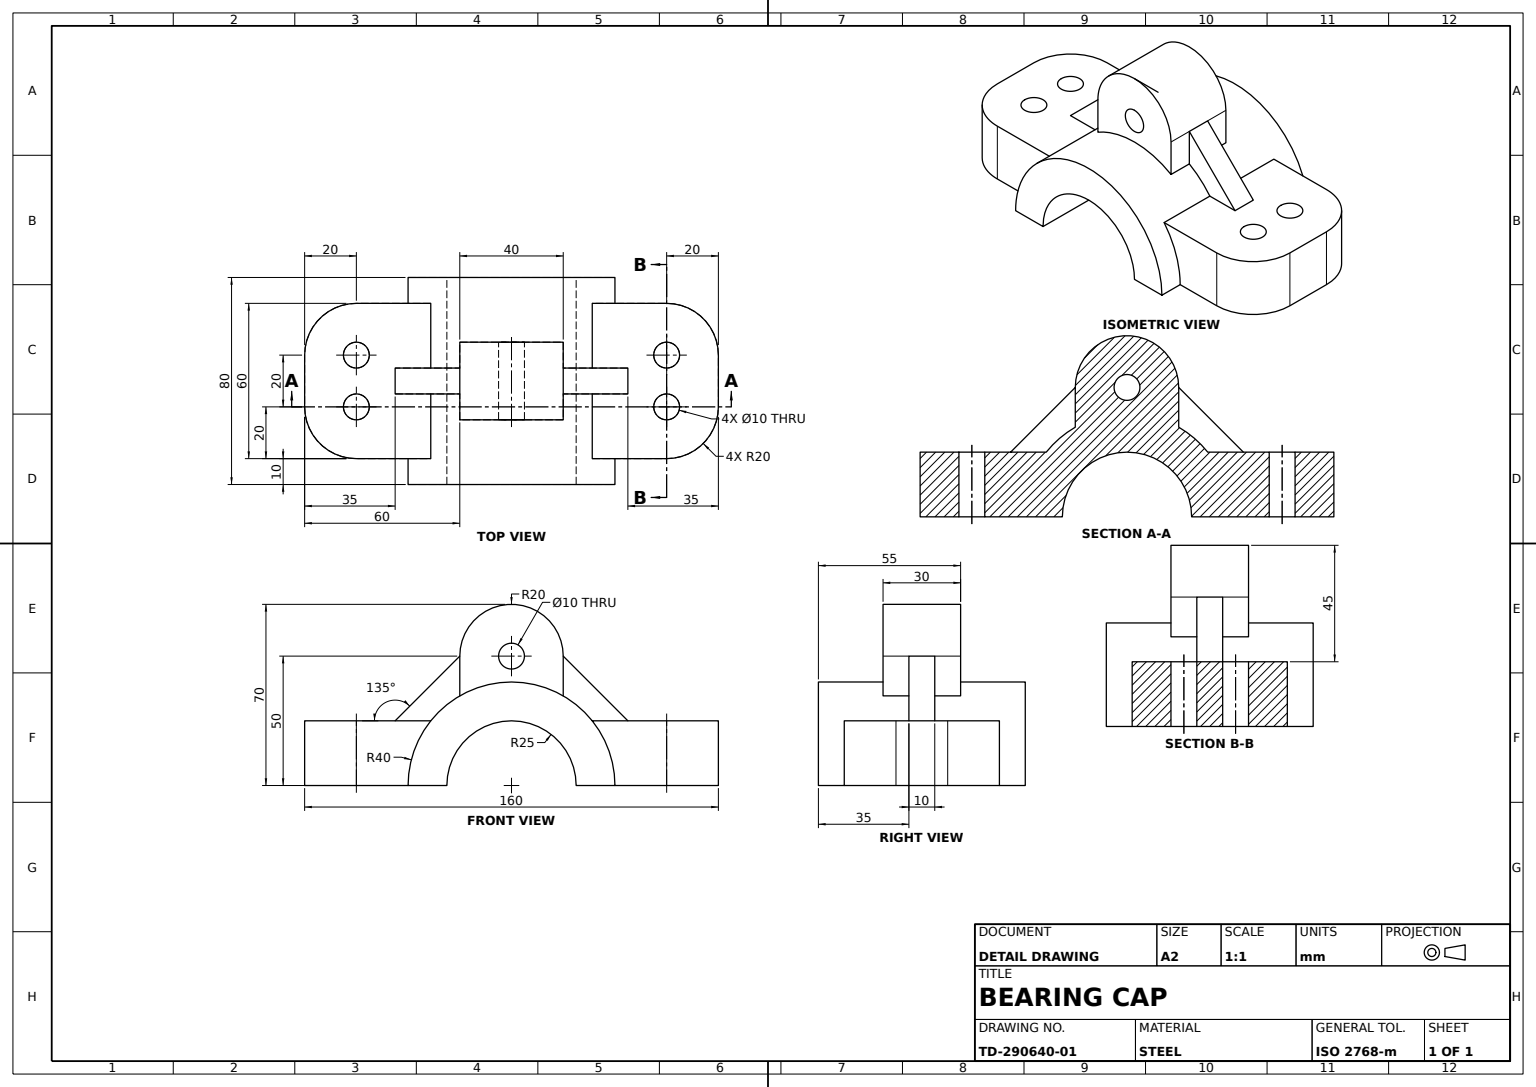
ISO-10303-21;
HEADER;
FILE_DESCRIPTION((''),'2;1');
FILE_NAME('','',(''),(''),'','','');
FILE_SCHEMA(('AUTOMOTIVE_DESIGN'));
ENDSEC;
DATA;
#1=APPLICATION_CONTEXT('');
#2=PRODUCT_CONTEXT('',#1,'mechanical');
#3=PRODUCT('','','',(#2));
#4=PRODUCT_DEFINITION_FORMATION('','',#3);
#5=PRODUCT_DEFINITION_CONTEXT('',#1,'design');
#6=PRODUCT_DEFINITION('','',#4,#5);
#7=PRODUCT_DEFINITION_SHAPE('','',#6);
#8=(LENGTH_UNIT()NAMED_UNIT(*)SI_UNIT(.MILLI.,.METRE.));
#9=(NAMED_UNIT(*)PLANE_ANGLE_UNIT()SI_UNIT($,.RADIAN.));
#10=(NAMED_UNIT(*)SI_UNIT($,.STERADIAN.)SOLID_ANGLE_UNIT());
#11=UNCERTAINTY_MEASURE_WITH_UNIT(LENGTH_MEASURE(0.005),#8,'distance_accuracy_value','');
#12=(GEOMETRIC_REPRESENTATION_CONTEXT(3)GLOBAL_UNCERTAINTY_ASSIGNED_CONTEXT((#11))GLOBAL_UNIT_ASSIGNED_CONTEXT((#8,#9,#10))REPRESENTATION_CONTEXT('',''));
#13=CARTESIAN_POINT('',(80.,10.,25.));
#14=VERTEX_POINT('',#13);
#15=CARTESIAN_POINT('',(60.,30.,25.));
#16=VERTEX_POINT('',#15);
#17=CARTESIAN_POINT('',(60.,10.,25.));
#18=DIRECTION('',(0.,0.,1.));
#19=DIRECTION('',(1.,0.,0.));
#20=AXIS2_PLACEMENT_3D('',#17,#18,#19);
#21=CIRCLE('',#20,20.);
#22=EDGE_CURVE('',#14,#16,#21,.T.);
#23=ORIENTED_EDGE('',*,*,#22,.F.);
#24=CARTESIAN_POINT('',(80.,10.,0.));
#25=VERTEX_POINT('',#24);
#26=DIRECTION('',(0.,0.,-1.));
#27=VECTOR('',#26,1000.);
#28=LINE('',#13,#27);
#29=EDGE_CURVE('',#25,#14,#28,.F.);
#30=ORIENTED_EDGE('',*,*,#29,.F.);
#31=CARTESIAN_POINT('',(60.,30.,0.));
#32=VERTEX_POINT('',#31);
#33=CARTESIAN_POINT('',(60.,10.,0.));
#34=AXIS2_PLACEMENT_3D('',#33,#18,#19);
#35=CIRCLE('',#34,20.);
#36=EDGE_CURVE('',#32,#25,#35,.F.);
#37=ORIENTED_EDGE('',*,*,#36,.F.);
#38=LINE('',#15,#27);
#39=EDGE_CURVE('',#16,#32,#38,.T.);
#40=ORIENTED_EDGE('',*,*,#39,.F.);
#41=EDGE_LOOP('',(#23,#30,#37,#40));
#42=FACE_BOUND('',#41,.T.);
#43=DIRECTION('',(-1.,0.,0.));
#44=AXIS2_PLACEMENT_3D('',#17,#26,#43);
#45=CYLINDRICAL_SURFACE('',#44,20.);
#46=ADVANCED_FACE('',(#42),#45,.T.);
#47=CARTESIAN_POINT('',(-55.,10.,0.));
#48=VERTEX_POINT('',#47);
#49=CARTESIAN_POINT('',(-60.,10.,0.));
#50=AXIS2_PLACEMENT_3D('',#49,#18,#19);
#51=CIRCLE('',#50,5.);
#52=EDGE_CURVE('',#48,#48,#51,.T.);
#53=ORIENTED_EDGE('',*,*,#52,.F.);
#54=EDGE_LOOP('',(#53));
#55=FACE_BOUND('',#54,.T.);
#56=CARTESIAN_POINT('',(-65.,10.,25.));
#57=VERTEX_POINT('',#56);
#58=CARTESIAN_POINT('',(-60.,10.,25.));
#59=AXIS2_PLACEMENT_3D('',#58,#26,#43);
#60=CIRCLE('',#59,5.);
#61=EDGE_CURVE('',#57,#57,#60,.T.);
#62=ORIENTED_EDGE('',*,*,#61,.F.);
#63=EDGE_LOOP('',(#62));
#64=FACE_BOUND('',#63,.T.);
#65=CYLINDRICAL_SURFACE('',#59,5.);
#66=ADVANCED_FACE('',(#55,#64),#65,.F.);
#67=CARTESIAN_POINT('',(-20.,15.,50.));
#68=VERTEX_POINT('',#67);
#69=CARTESIAN_POINT('',(-20.,15.,34.641016));
#70=VERTEX_POINT('',#69);
#71=LINE('',#67,#27);
#72=EDGE_CURVE('',#68,#70,#71,.T.);
#73=ORIENTED_EDGE('',*,*,#72,.T.);
#74=CARTESIAN_POINT('',(-20.,5.,34.641016));
#75=VERTEX_POINT('',#74);
#76=CARTESIAN_POINT('',(-20.,-40.,34.641016));
#77=DIRECTION('',(0.,1.,0.));
#78=VECTOR('',#77,1000.);
#79=LINE('',#76,#78);
#80=EDGE_CURVE('',#70,#75,#79,.F.);
#81=ORIENTED_EDGE('',*,*,#80,.T.);
#82=CARTESIAN_POINT('',(-20.,5.,50.));
#83=VERTEX_POINT('',#82);
#84=CARTESIAN_POINT('',(-20.,5.,0.));
#85=VECTOR('',#18,1000.);
#86=LINE('',#84,#85);
#87=EDGE_CURVE('',#75,#83,#86,.T.);
#88=ORIENTED_EDGE('',*,*,#87,.T.);
#89=CARTESIAN_POINT('',(-20.,-15.,50.));
#90=LINE('',#89,#78);
#91=EDGE_CURVE('',#83,#68,#90,.T.);
#92=ORIENTED_EDGE('',*,*,#91,.T.);
#93=EDGE_LOOP('',(#73,#81,#88,#92));
#94=FACE_BOUND('',#93,.T.);
#95=AXIS2_PLACEMENT_3D('',#89,#19,#26);
#96=PLANE('',#95);
#97=ADVANCED_FACE('',(#94),#96,.F.);
#98=CARTESIAN_POINT('',(45.,5.,25.));
#99=VERTEX_POINT('',#98);
#100=CARTESIAN_POINT('',(31.22499,5.,25.));
#101=VERTEX_POINT('',#100);
#102=CARTESIAN_POINT('',(0.,5.,25.));
#103=VECTOR('',#43,1000.);
#104=LINE('',#102,#103);
#105=EDGE_CURVE('',#99,#101,#104,.T.);
#106=ORIENTED_EDGE('',*,*,#105,.T.);
#107=CARTESIAN_POINT('',(20.,5.,34.641016));
#108=VERTEX_POINT('',#107);
#109=CARTESIAN_POINT('',(0.,5.,0.));
#110=AXIS2_PLACEMENT_3D('',#109,#77,#18);
#111=CIRCLE('',#110,40.);
#112=EDGE_CURVE('',#108,#101,#111,.T.);
#113=ORIENTED_EDGE('',*,*,#112,.F.);
#114=CARTESIAN_POINT('',(20.,5.,50.));
#115=VERTEX_POINT('',#114);
#116=CARTESIAN_POINT('',(20.,5.,0.));
#117=LINE('',#116,#85);
#118=EDGE_CURVE('',#108,#115,#117,.T.);
#119=ORIENTED_EDGE('',*,*,#118,.T.);
#120=DIRECTION('',(0.707106781,0.,-0.707106781));
#121=VECTOR('',#120,1000.);
#122=LINE('',#114,#121);
#123=EDGE_CURVE('',#115,#99,#122,.T.);
#124=ORIENTED_EDGE('',*,*,#123,.T.);
#125=EDGE_LOOP('',(#106,#113,#119,#124));
#126=FACE_BOUND('',#125,.T.);
#127=PLANE('',#110);
#128=ADVANCED_FACE('',(#126),#127,.T.);
#129=CARTESIAN_POINT('',(-65.,-10.,25.));
#130=VERTEX_POINT('',#129);
#131=CARTESIAN_POINT('',(-60.,-10.,25.));
#132=AXIS2_PLACEMENT_3D('',#131,#26,#43);
#133=CIRCLE('',#132,5.);
#134=EDGE_CURVE('',#130,#130,#133,.T.);
#135=ORIENTED_EDGE('',*,*,#134,.F.);
#136=EDGE_LOOP('',(#135));
#137=FACE_BOUND('',#136,.T.);
#138=CARTESIAN_POINT('',(-55.,-10.,0.));
#139=VERTEX_POINT('',#138);
#140=CARTESIAN_POINT('',(-60.,-10.,0.));
#141=AXIS2_PLACEMENT_3D('',#140,#18,#19);
#142=CIRCLE('',#141,5.);
#143=EDGE_CURVE('',#139,#139,#142,.T.);
#144=ORIENTED_EDGE('',*,*,#143,.F.);
#145=EDGE_LOOP('',(#144));
#146=FACE_BOUND('',#145,.T.);
#147=CYLINDRICAL_SURFACE('',#132,5.);
#148=ADVANCED_FACE('',(#137,#146),#147,.F.);
#149=CARTESIAN_POINT('',(-45.,5.,25.));
#150=VERTEX_POINT('',#149);
#151=CARTESIAN_POINT('',(-31.22499,5.,25.));
#152=VERTEX_POINT('',#151);
#153=VECTOR('',#19,1000.);
#154=LINE('',#102,#153);
#155=EDGE_CURVE('',#150,#152,#154,.T.);
#156=ORIENTED_EDGE('',*,*,#155,.F.);
#157=DIRECTION('',(-0.707106781,0.,-0.707106781));
#158=VECTOR('',#157,1000.);
#159=LINE('',#82,#158);
#160=EDGE_CURVE('',#83,#150,#159,.T.);
#161=ORIENTED_EDGE('',*,*,#160,.F.);
#162=ORIENTED_EDGE('',*,*,#87,.F.);
#163=DIRECTION('',(0.,-1.,0.));
#164=AXIS2_PLACEMENT_3D('',#109,#163,#26);
#165=CIRCLE('',#164,40.);
#166=EDGE_CURVE('',#75,#152,#165,.T.);
#167=ORIENTED_EDGE('',*,*,#166,.T.);
#168=EDGE_LOOP('',(#156,#161,#162,#167));
#169=FACE_BOUND('',#168,.T.);
#170=PLANE('',#164);
#171=ADVANCED_FACE('',(#169),#170,.F.);
#172=CARTESIAN_POINT('',(25.,40.,0.));
#173=VERTEX_POINT('',#172);
#174=CARTESIAN_POINT('',(40.,40.,0.));
#175=VERTEX_POINT('',#174);
#176=CARTESIAN_POINT('',(0.,40.,0.));
#177=LINE('',#176,#153);
#178=EDGE_CURVE('',#173,#175,#177,.T.);
#179=ORIENTED_EDGE('',*,*,#178,.F.);
#180=CARTESIAN_POINT('',(-25.,40.,0.));
#181=VERTEX_POINT('',#180);
#182=AXIS2_PLACEMENT_3D('',#176,#163,#26);
#183=CIRCLE('',#182,25.);
#184=EDGE_CURVE('',#173,#181,#183,.T.);
#185=ORIENTED_EDGE('',*,*,#184,.T.);
#186=CARTESIAN_POINT('',(-40.,40.,0.));
#187=VERTEX_POINT('',#186);
#188=EDGE_CURVE('',#187,#181,#177,.T.);
#189=ORIENTED_EDGE('',*,*,#188,.F.);
#190=AXIS2_PLACEMENT_3D('',#176,#163,#19);
#191=CIRCLE('',#190,40.);
#192=EDGE_CURVE('',#175,#187,#191,.T.);
#193=ORIENTED_EDGE('',*,*,#192,.F.);
#194=EDGE_LOOP('',(#179,#185,#189,#193));
#195=FACE_BOUND('',#194,.T.);
#196=PLANE('',#182);
#197=ADVANCED_FACE('',(#195),#196,.F.);
#198=CARTESIAN_POINT('',(80.,-10.,0.));
#199=VERTEX_POINT('',#198);
#200=CARTESIAN_POINT('',(60.,-30.,0.));
#201=VERTEX_POINT('',#200);
#202=CARTESIAN_POINT('',(60.,-10.,0.));
#203=AXIS2_PLACEMENT_3D('',#202,#18,#19);
#204=CIRCLE('',#203,20.);
#205=EDGE_CURVE('',#199,#201,#204,.F.);
#206=ORIENTED_EDGE('',*,*,#205,.F.);
#207=CARTESIAN_POINT('',(80.,-10.,25.));
#208=VERTEX_POINT('',#207);
#209=LINE('',#207,#27);
#210=EDGE_CURVE('',#208,#199,#209,.T.);
#211=ORIENTED_EDGE('',*,*,#210,.F.);
#212=CARTESIAN_POINT('',(60.,-30.,25.));
#213=VERTEX_POINT('',#212);
#214=CARTESIAN_POINT('',(60.,-10.,25.));
#215=AXIS2_PLACEMENT_3D('',#214,#18,#19);
#216=CIRCLE('',#215,20.);
#217=EDGE_CURVE('',#213,#208,#216,.T.);
#218=ORIENTED_EDGE('',*,*,#217,.F.);
#219=LINE('',#212,#27);
#220=EDGE_CURVE('',#201,#213,#219,.F.);
#221=ORIENTED_EDGE('',*,*,#220,.F.);
#222=EDGE_LOOP('',(#206,#211,#218,#221));
#223=FACE_BOUND('',#222,.T.);
#224=AXIS2_PLACEMENT_3D('',#214,#26,#43);
#225=CYLINDRICAL_SURFACE('',#224,20.);
#226=ADVANCED_FACE('',(#223),#225,.T.);
#227=ORIENTED_EDGE('',*,*,#61,.T.);
#228=EDGE_LOOP('',(#227));
#229=FACE_BOUND('',#228,.T.);
#230=ORIENTED_EDGE('',*,*,#134,.T.);
#231=EDGE_LOOP('',(#230));
#232=FACE_BOUND('',#231,.T.);
#233=CARTESIAN_POINT('',(-80.,10.,25.));
#234=VERTEX_POINT('',#233);
#235=CARTESIAN_POINT('',(-80.,-10.,25.));
#236=VERTEX_POINT('',#235);
#237=CARTESIAN_POINT('',(-80.,30.,25.));
#238=VECTOR('',#163,1000.);
#239=LINE('',#237,#238);
#240=EDGE_CURVE('',#234,#236,#239,.T.);
#241=ORIENTED_EDGE('',*,*,#240,.T.);
#242=CARTESIAN_POINT('',(-60.,-30.,25.));
#243=VERTEX_POINT('',#242);
#244=AXIS2_PLACEMENT_3D('',#131,#18,#19);
#245=CIRCLE('',#244,20.);
#246=EDGE_CURVE('',#236,#243,#245,.T.);
#247=ORIENTED_EDGE('',*,*,#246,.T.);
#248=CARTESIAN_POINT('',(-31.22499,-30.,25.));
#249=VERTEX_POINT('',#248);
#250=CARTESIAN_POINT('',(-80.,-30.,25.));
#251=LINE('',#250,#153);
#252=EDGE_CURVE('',#243,#249,#251,.T.);
#253=ORIENTED_EDGE('',*,*,#252,.T.);
#254=CARTESIAN_POINT('',(-31.22499,-5.,25.));
#255=VERTEX_POINT('',#254);
#256=CARTESIAN_POINT('',(-31.22499,-40.,25.));
#257=LINE('',#256,#78);
#258=EDGE_CURVE('',#255,#249,#257,.F.);
#259=ORIENTED_EDGE('',*,*,#258,.F.);
#260=CARTESIAN_POINT('',(-45.,-5.,25.));
#261=VERTEX_POINT('',#260);
#262=CARTESIAN_POINT('',(0.,-5.,25.));
#263=LINE('',#262,#153);
#264=EDGE_CURVE('',#261,#255,#263,.T.);
#265=ORIENTED_EDGE('',*,*,#264,.F.);
#266=CARTESIAN_POINT('',(-45.,0.,25.));
#267=LINE('',#266,#78);
#268=EDGE_CURVE('',#261,#150,#267,.T.);
#269=ORIENTED_EDGE('',*,*,#268,.T.);
#270=ORIENTED_EDGE('',*,*,#155,.T.);
#271=CARTESIAN_POINT('',(-31.22499,30.,25.));
#272=VERTEX_POINT('',#271);
#273=EDGE_CURVE('',#272,#152,#257,.F.);
#274=ORIENTED_EDGE('',*,*,#273,.F.);
#275=CARTESIAN_POINT('',(-60.,30.,25.));
#276=VERTEX_POINT('',#275);
#277=CARTESIAN_POINT('',(80.,30.,25.));
#278=LINE('',#277,#103);
#279=EDGE_CURVE('',#272,#276,#278,.T.);
#280=ORIENTED_EDGE('',*,*,#279,.T.);
#281=AXIS2_PLACEMENT_3D('',#58,#18,#19);
#282=CIRCLE('',#281,20.);
#283=EDGE_CURVE('',#276,#234,#282,.T.);
#284=ORIENTED_EDGE('',*,*,#283,.T.);
#285=EDGE_LOOP('',(#241,#247,#253,#259,#265,#269,#270,#274,#280,#284));
#286=FACE_BOUND('',#285,.T.);
#287=CARTESIAN_POINT('',(0.,0.,25.));
#288=AXIS2_PLACEMENT_3D('',#287,#18,#19);
#289=PLANE('',#288);
#290=ADVANCED_FACE('',(#229,#232,#286),#289,.T.);
#291=CARTESIAN_POINT('',(65.,-10.,0.));
#292=VERTEX_POINT('',#291);
#293=CIRCLE('',#203,5.);
#294=EDGE_CURVE('',#292,#292,#293,.T.);
#295=ORIENTED_EDGE('',*,*,#294,.F.);
#296=EDGE_LOOP('',(#295));
#297=FACE_BOUND('',#296,.T.);
#298=CARTESIAN_POINT('',(55.,-10.,25.));
#299=VERTEX_POINT('',#298);
#300=CIRCLE('',#224,5.);
#301=EDGE_CURVE('',#299,#299,#300,.T.);
#302=ORIENTED_EDGE('',*,*,#301,.F.);
#303=EDGE_LOOP('',(#302));
#304=FACE_BOUND('',#303,.T.);
#305=CYLINDRICAL_SURFACE('',#224,5.);
#306=ADVANCED_FACE('',(#297,#304),#305,.F.);
#307=CARTESIAN_POINT('',(-60.,30.,0.));
#308=VERTEX_POINT('',#307);
#309=LINE('',#275,#27);
#310=EDGE_CURVE('',#308,#276,#309,.F.);
#311=ORIENTED_EDGE('',*,*,#310,.T.);
#312=ORIENTED_EDGE('',*,*,#279,.F.);
#313=CARTESIAN_POINT('',(-40.,30.,0.));
#314=VERTEX_POINT('',#313);
#315=CARTESIAN_POINT('',(0.,30.,0.));
#316=AXIS2_PLACEMENT_3D('',#315,#163,#26);
#317=CIRCLE('',#316,40.);
#318=EDGE_CURVE('',#272,#314,#317,.T.);
#319=ORIENTED_EDGE('',*,*,#318,.T.);
#320=CARTESIAN_POINT('',(80.,30.,0.));
#321=LINE('',#320,#103);
#322=EDGE_CURVE('',#314,#308,#321,.T.);
#323=ORIENTED_EDGE('',*,*,#322,.T.);
#324=EDGE_LOOP('',(#311,#312,#319,#323));
#325=FACE_BOUND('',#324,.T.);
#326=AXIS2_PLACEMENT_3D('',#277,#163,#26);
#327=PLANE('',#326);
#328=ADVANCED_FACE('',(#325),#327,.F.);
#329=CARTESIAN_POINT('',(0.,-15.,55.));
#330=VERTEX_POINT('',#329);
#331=CARTESIAN_POINT('',(0.,-15.,50.));
#332=AXIS2_PLACEMENT_3D('',#331,#77,#18);
#333=CIRCLE('',#332,5.);
#334=EDGE_CURVE('',#330,#330,#333,.T.);
#335=ORIENTED_EDGE('',*,*,#334,.T.);
#336=EDGE_LOOP('',(#335));
#337=FACE_BOUND('',#336,.T.);
#338=CARTESIAN_POINT('',(20.,-15.,34.641016));
#339=VERTEX_POINT('',#338);
#340=CARTESIAN_POINT('',(-20.,-15.,34.641016));
#341=VERTEX_POINT('',#340);
#342=CARTESIAN_POINT('',(0.,-15.,0.));
#343=AXIS2_PLACEMENT_3D('',#342,#163,#26);
#344=CIRCLE('',#343,40.);
#345=EDGE_CURVE('',#339,#341,#344,.T.);
#346=ORIENTED_EDGE('',*,*,#345,.F.);
#347=CARTESIAN_POINT('',(20.,-15.,50.));
#348=VERTEX_POINT('',#347);
#349=CARTESIAN_POINT('',(20.,-15.,0.));
#350=LINE('',#349,#85);
#351=EDGE_CURVE('',#339,#348,#350,.T.);
#352=ORIENTED_EDGE('',*,*,#351,.T.);
#353=VERTEX_POINT('',#89);
#354=AXIS2_PLACEMENT_3D('',#331,#163,#19);
#355=CIRCLE('',#354,20.);
#356=EDGE_CURVE('',#348,#353,#355,.T.);
#357=ORIENTED_EDGE('',*,*,#356,.T.);
#358=LINE('',#89,#27);
#359=EDGE_CURVE('',#353,#341,#358,.T.);
#360=ORIENTED_EDGE('',*,*,#359,.T.);
#361=EDGE_LOOP('',(#346,#352,#357,#360));
#362=FACE_BOUND('',#361,.T.);
#363=AXIS2_PLACEMENT_3D('',#331,#163,#26);
#364=PLANE('',#363);
#365=ADVANCED_FACE('',(#337,#362),#364,.T.);
#366=CARTESIAN_POINT('',(55.,10.,25.));
#367=VERTEX_POINT('',#366);
#368=CIRCLE('',#44,5.);
#369=EDGE_CURVE('',#367,#367,#368,.T.);
#370=ORIENTED_EDGE('',*,*,#369,.F.);
#371=EDGE_LOOP('',(#370));
#372=FACE_BOUND('',#371,.T.);
#373=CARTESIAN_POINT('',(65.,10.,0.));
#374=VERTEX_POINT('',#373);
#375=CIRCLE('',#34,5.);
#376=EDGE_CURVE('',#374,#374,#375,.T.);
#377=ORIENTED_EDGE('',*,*,#376,.F.);
#378=EDGE_LOOP('',(#377));
#379=FACE_BOUND('',#378,.T.);
#380=CYLINDRICAL_SURFACE('',#44,5.);
#381=ADVANCED_FACE('',(#372,#379),#380,.F.);
#382=CARTESIAN_POINT('',(45.,-5.,25.));
#383=VERTEX_POINT('',#382);
#384=CARTESIAN_POINT('',(45.,0.,25.));
#385=LINE('',#384,#78);
#386=EDGE_CURVE('',#383,#99,#385,.T.);
#387=ORIENTED_EDGE('',*,*,#386,.T.);
#388=ORIENTED_EDGE('',*,*,#123,.F.);
#389=CARTESIAN_POINT('',(20.,-5.,50.));
#390=VERTEX_POINT('',#389);
#391=LINE('',#389,#78);
#392=EDGE_CURVE('',#390,#115,#391,.T.);
#393=ORIENTED_EDGE('',*,*,#392,.F.);
#394=LINE('',#389,#121);
#395=EDGE_CURVE('',#390,#383,#394,.T.);
#396=ORIENTED_EDGE('',*,*,#395,.T.);
#397=EDGE_LOOP('',(#387,#388,#393,#396));
#398=FACE_BOUND('',#397,.T.);
#399=DIRECTION('',(0.707106781,0.,0.707106781));
#400=AXIS2_PLACEMENT_3D('',#389,#399,#120);
#401=PLANE('',#400);
#402=ADVANCED_FACE('',(#398),#401,.T.);
#403=CARTESIAN_POINT('',(-60.,-30.,0.));
#404=VERTEX_POINT('',#403);
#405=CARTESIAN_POINT('',(-80.,-10.,0.));
#406=VERTEX_POINT('',#405);
#407=CIRCLE('',#141,20.);
#408=EDGE_CURVE('',#404,#406,#407,.F.);
#409=ORIENTED_EDGE('',*,*,#408,.F.);
#410=LINE('',#242,#27);
#411=EDGE_CURVE('',#243,#404,#410,.T.);
#412=ORIENTED_EDGE('',*,*,#411,.F.);
#413=ORIENTED_EDGE('',*,*,#246,.F.);
#414=LINE('',#235,#27);
#415=EDGE_CURVE('',#406,#236,#414,.F.);
#416=ORIENTED_EDGE('',*,*,#415,.F.);
#417=EDGE_LOOP('',(#409,#412,#413,#416));
#418=FACE_BOUND('',#417,.T.);
#419=CYLINDRICAL_SURFACE('',#132,20.);
#420=ADVANCED_FACE('',(#418),#419,.T.);
#421=ORIENTED_EDGE('',*,*,#240,.F.);
#422=CARTESIAN_POINT('',(-80.,10.,0.));
#423=VERTEX_POINT('',#422);
#424=LINE('',#233,#27);
#425=EDGE_CURVE('',#234,#423,#424,.T.);
#426=ORIENTED_EDGE('',*,*,#425,.T.);
#427=CARTESIAN_POINT('',(-80.,30.,0.));
#428=LINE('',#427,#238);
#429=EDGE_CURVE('',#423,#406,#428,.T.);
#430=ORIENTED_EDGE('',*,*,#429,.T.);
#431=ORIENTED_EDGE('',*,*,#415,.T.);
#432=EDGE_LOOP('',(#421,#426,#430,#431));
#433=FACE_BOUND('',#432,.T.);
#434=AXIS2_PLACEMENT_3D('',#237,#19,#26);
#435=PLANE('',#434);
#436=ADVANCED_FACE('',(#433),#435,.F.);
#437=ORIENTED_EDGE('',*,*,#264,.T.);
#438=CARTESIAN_POINT('',(-20.,-5.,34.641016));
#439=VERTEX_POINT('',#438);
#440=CARTESIAN_POINT('',(0.,-5.,0.));
#441=AXIS2_PLACEMENT_3D('',#440,#163,#26);
#442=CIRCLE('',#441,40.);
#443=EDGE_CURVE('',#439,#255,#442,.T.);
#444=ORIENTED_EDGE('',*,*,#443,.F.);
#445=CARTESIAN_POINT('',(-20.,-5.,50.));
#446=VERTEX_POINT('',#445);
#447=CARTESIAN_POINT('',(-20.,-5.,0.));
#448=LINE('',#447,#85);
#449=EDGE_CURVE('',#439,#446,#448,.T.);
#450=ORIENTED_EDGE('',*,*,#449,.T.);
#451=LINE('',#445,#158);
#452=EDGE_CURVE('',#446,#261,#451,.T.);
#453=ORIENTED_EDGE('',*,*,#452,.T.);
#454=EDGE_LOOP('',(#437,#444,#450,#453));
#455=FACE_BOUND('',#454,.T.);
#456=PLANE('',#441);
#457=ADVANCED_FACE('',(#455),#456,.T.);
#458=ORIENTED_EDGE('',*,*,#334,.F.);
#459=EDGE_LOOP('',(#458));
#460=FACE_BOUND('',#459,.T.);
#461=CARTESIAN_POINT('',(0.,15.,45.));
#462=VERTEX_POINT('',#461);
#463=CARTESIAN_POINT('',(0.,15.,50.));
#464=AXIS2_PLACEMENT_3D('',#463,#163,#26);
#465=CIRCLE('',#464,5.);
#466=EDGE_CURVE('',#462,#462,#465,.T.);
#467=ORIENTED_EDGE('',*,*,#466,.F.);
#468=EDGE_LOOP('',(#467));
#469=FACE_BOUND('',#468,.T.);
#470=CYLINDRICAL_SURFACE('',#332,5.);
#471=ADVANCED_FACE('',(#460,#469),#470,.F.);
#472=LINE('',#347,#78);
#473=EDGE_CURVE('',#348,#390,#472,.T.);
#474=ORIENTED_EDGE('',*,*,#473,.F.);
#475=ORIENTED_EDGE('',*,*,#351,.F.);
#476=CARTESIAN_POINT('',(20.,-5.,34.641016));
#477=VERTEX_POINT('',#476);
#478=CARTESIAN_POINT('',(20.,-40.,34.641016));
#479=LINE('',#478,#78);
#480=EDGE_CURVE('',#339,#477,#479,.T.);
#481=ORIENTED_EDGE('',*,*,#480,.T.);
#482=CARTESIAN_POINT('',(20.,-5.,0.));
#483=LINE('',#482,#85);
#484=EDGE_CURVE('',#477,#390,#483,.T.);
#485=ORIENTED_EDGE('',*,*,#484,.T.);
#486=EDGE_LOOP('',(#474,#475,#481,#485));
#487=FACE_BOUND('',#486,.T.);
#488=AXIS2_PLACEMENT_3D('',#349,#43,#18);
#489=PLANE('',#488);
#490=ADVANCED_FACE('',(#487),#489,.F.);
#491=EDGE_CURVE('',#353,#446,#90,.T.);
#492=ORIENTED_EDGE('',*,*,#491,.T.);
#493=ORIENTED_EDGE('',*,*,#449,.F.);
#494=EDGE_CURVE('',#439,#341,#79,.F.);
#495=ORIENTED_EDGE('',*,*,#494,.T.);
#496=ORIENTED_EDGE('',*,*,#359,.F.);
#497=EDGE_LOOP('',(#492,#493,#495,#496));
#498=FACE_BOUND('',#497,.T.);
#499=ADVANCED_FACE('',(#498),#96,.F.);
#500=ORIENTED_EDGE('',*,*,#184,.F.);
#501=CARTESIAN_POINT('',(25.,-40.,0.));
#502=VERTEX_POINT('',#501);
#503=LINE('',#501,#78);
#504=EDGE_CURVE('',#502,#173,#503,.T.);
#505=ORIENTED_EDGE('',*,*,#504,.F.);
#506=CARTESIAN_POINT('',(-25.,-40.,0.));
#507=VERTEX_POINT('',#506);
#508=CARTESIAN_POINT('',(0.,-40.,0.));
#509=AXIS2_PLACEMENT_3D('',#508,#77,#18);
#510=CIRCLE('',#509,25.);
#511=EDGE_CURVE('',#507,#502,#510,.T.);
#512=ORIENTED_EDGE('',*,*,#511,.F.);
#513=LINE('',#506,#78);
#514=EDGE_CURVE('',#181,#507,#513,.F.);
#515=ORIENTED_EDGE('',*,*,#514,.F.);
#516=EDGE_LOOP('',(#500,#505,#512,#515));
#517=FACE_BOUND('',#516,.T.);
#518=CYLINDRICAL_SURFACE('',#509,25.);
#519=ADVANCED_FACE('',(#517),#518,.F.);
#520=ORIENTED_EDGE('',*,*,#484,.F.);
#521=CARTESIAN_POINT('',(31.22499,-5.,25.));
#522=VERTEX_POINT('',#521);
#523=AXIS2_PLACEMENT_3D('',#440,#77,#18);
#524=CIRCLE('',#523,40.);
#525=EDGE_CURVE('',#477,#522,#524,.T.);
#526=ORIENTED_EDGE('',*,*,#525,.T.);
#527=LINE('',#262,#103);
#528=EDGE_CURVE('',#383,#522,#527,.T.);
#529=ORIENTED_EDGE('',*,*,#528,.F.);
#530=ORIENTED_EDGE('',*,*,#395,.F.);
#531=EDGE_LOOP('',(#520,#526,#529,#530));
#532=FACE_BOUND('',#531,.T.);
#533=PLANE('',#523);
#534=ADVANCED_FACE('',(#532),#533,.F.);
#535=ORIENTED_EDGE('',*,*,#160,.T.);
#536=ORIENTED_EDGE('',*,*,#268,.F.);
#537=ORIENTED_EDGE('',*,*,#452,.F.);
#538=LINE('',#445,#78);
#539=EDGE_CURVE('',#446,#83,#538,.T.);
#540=ORIENTED_EDGE('',*,*,#539,.T.);
#541=EDGE_LOOP('',(#535,#536,#537,#540));
#542=FACE_BOUND('',#541,.T.);
#543=AXIS2_PLACEMENT_3D('',#445,#120,#157);
#544=PLANE('',#543);
#545=ADVANCED_FACE('',(#542),#544,.F.);
#546=CARTESIAN_POINT('',(-40.,-30.,0.));
#547=VERTEX_POINT('',#546);
#548=CARTESIAN_POINT('',(0.,-30.,0.));
#549=AXIS2_PLACEMENT_3D('',#548,#77,#18);
#550=CIRCLE('',#549,40.);
#551=EDGE_CURVE('',#547,#249,#550,.T.);
#552=ORIENTED_EDGE('',*,*,#551,.F.);
#553=CARTESIAN_POINT('',(-40.,-40.,0.));
#554=VERTEX_POINT('',#553);
#555=LINE('',#553,#78);
#556=EDGE_CURVE('',#554,#547,#555,.T.);
#557=ORIENTED_EDGE('',*,*,#556,.F.);
#558=CARTESIAN_POINT('',(40.,-40.,0.));
#559=VERTEX_POINT('',#558);
#560=AXIS2_PLACEMENT_3D('',#508,#163,#19);
#561=CIRCLE('',#560,40.);
#562=EDGE_CURVE('',#559,#554,#561,.T.);
#563=ORIENTED_EDGE('',*,*,#562,.F.);
#564=CARTESIAN_POINT('',(40.,-30.,0.));
#565=VERTEX_POINT('',#564);
#566=LINE('',#558,#78);
#567=EDGE_CURVE('',#565,#559,#566,.F.);
#568=ORIENTED_EDGE('',*,*,#567,.F.);
#569=CARTESIAN_POINT('',(31.22499,-30.,25.));
#570=VERTEX_POINT('',#569);
#571=EDGE_CURVE('',#570,#565,#550,.T.);
#572=ORIENTED_EDGE('',*,*,#571,.F.);
#573=CARTESIAN_POINT('',(31.22499,-40.,25.));
#574=LINE('',#573,#78);
#575=EDGE_CURVE('',#570,#522,#574,.T.);
#576=ORIENTED_EDGE('',*,*,#575,.T.);
#577=ORIENTED_EDGE('',*,*,#525,.F.);
#578=ORIENTED_EDGE('',*,*,#480,.F.);
#579=ORIENTED_EDGE('',*,*,#345,.T.);
#580=ORIENTED_EDGE('',*,*,#494,.F.);
#581=ORIENTED_EDGE('',*,*,#443,.T.);
#582=ORIENTED_EDGE('',*,*,#258,.T.);
#583=EDGE_LOOP('',(#552,#557,#563,#568,#572,#576,#577,#578,#579,#580,#581,#582));
#584=FACE_BOUND('',#583,.T.);
#585=CYLINDRICAL_SURFACE('',#509,40.);
#586=ADVANCED_FACE('',(#584),#585,.T.);
#587=ORIENTED_EDGE('',*,*,#318,.F.);
#588=ORIENTED_EDGE('',*,*,#273,.T.);
#589=ORIENTED_EDGE('',*,*,#166,.F.);
#590=ORIENTED_EDGE('',*,*,#80,.F.);
#591=CARTESIAN_POINT('',(20.,15.,34.641016));
#592=VERTEX_POINT('',#591);
#593=CARTESIAN_POINT('',(0.,15.,0.));
#594=AXIS2_PLACEMENT_3D('',#593,#163,#26);
#595=CIRCLE('',#594,40.);
#596=EDGE_CURVE('',#592,#70,#595,.T.);
#597=ORIENTED_EDGE('',*,*,#596,.F.);
#598=EDGE_CURVE('',#108,#592,#479,.T.);
#599=ORIENTED_EDGE('',*,*,#598,.F.);
#600=ORIENTED_EDGE('',*,*,#112,.T.);
#601=CARTESIAN_POINT('',(31.22499,30.,25.));
#602=VERTEX_POINT('',#601);
#603=EDGE_CURVE('',#101,#602,#574,.T.);
#604=ORIENTED_EDGE('',*,*,#603,.T.);
#605=CARTESIAN_POINT('',(40.,30.,0.));
#606=VERTEX_POINT('',#605);
#607=EDGE_CURVE('',#606,#602,#317,.T.);
#608=ORIENTED_EDGE('',*,*,#607,.F.);
#609=EDGE_CURVE('',#175,#606,#566,.F.);
#610=ORIENTED_EDGE('',*,*,#609,.F.);
#611=ORIENTED_EDGE('',*,*,#192,.T.);
#612=EDGE_CURVE('',#314,#187,#555,.T.);
#613=ORIENTED_EDGE('',*,*,#612,.F.);
#614=EDGE_LOOP('',(#587,#588,#589,#590,#597,#599,#600,#604,#608,#610,#611,#613));
#615=FACE_BOUND('',#614,.T.);
#616=ADVANCED_FACE('',(#615),#585,.T.);
#617=CARTESIAN_POINT('',(20.,15.,50.));
#618=VERTEX_POINT('',#617);
#619=AXIS2_PLACEMENT_3D('',#463,#163,#19);
#620=CIRCLE('',#619,20.);
#621=EDGE_CURVE('',#618,#68,#620,.T.);
#622=ORIENTED_EDGE('',*,*,#621,.T.);
#623=ORIENTED_EDGE('',*,*,#91,.F.);
#624=ORIENTED_EDGE('',*,*,#539,.F.);
#625=ORIENTED_EDGE('',*,*,#491,.F.);
#626=ORIENTED_EDGE('',*,*,#356,.F.);
#627=ORIENTED_EDGE('',*,*,#473,.T.);
#628=ORIENTED_EDGE('',*,*,#392,.T.);
#629=EDGE_CURVE('',#115,#618,#472,.T.);
#630=ORIENTED_EDGE('',*,*,#629,.T.);
#631=EDGE_LOOP('',(#622,#623,#624,#625,#626,#627,#628,#630));
#632=FACE_BOUND('',#631,.T.);
#633=CYLINDRICAL_SURFACE('',#332,20.);
#634=ADVANCED_FACE('',(#632),#633,.T.);
#635=ORIENTED_EDGE('',*,*,#220,.T.);
#636=EDGE_CURVE('',#570,#213,#251,.T.);
#637=ORIENTED_EDGE('',*,*,#636,.F.);
#638=ORIENTED_EDGE('',*,*,#571,.T.);
#639=CARTESIAN_POINT('',(-80.,-30.,0.));
#640=LINE('',#639,#153);
#641=EDGE_CURVE('',#565,#201,#640,.T.);
#642=ORIENTED_EDGE('',*,*,#641,.T.);
#643=EDGE_LOOP('',(#635,#637,#638,#642));
#644=FACE_BOUND('',#643,.T.);
#645=AXIS2_PLACEMENT_3D('',#250,#77,#18);
#646=PLANE('',#645);
#647=ADVANCED_FACE('',(#644),#646,.F.);
#648=ORIENTED_EDGE('',*,*,#294,.T.);
#649=EDGE_LOOP('',(#648));
#650=FACE_BOUND('',#649,.T.);
#651=ORIENTED_EDGE('',*,*,#376,.T.);
#652=EDGE_LOOP('',(#651));
#653=FACE_BOUND('',#652,.T.);
#654=EDGE_CURVE('',#32,#606,#321,.T.);
#655=ORIENTED_EDGE('',*,*,#654,.F.);
#656=ORIENTED_EDGE('',*,*,#36,.T.);
#657=CARTESIAN_POINT('',(80.,-30.,0.));
#658=LINE('',#657,#78);
#659=EDGE_CURVE('',#199,#25,#658,.T.);
#660=ORIENTED_EDGE('',*,*,#659,.F.);
#661=ORIENTED_EDGE('',*,*,#205,.T.);
#662=ORIENTED_EDGE('',*,*,#641,.F.);
#663=ORIENTED_EDGE('',*,*,#567,.T.);
#664=LINE('',#508,#153);
#665=EDGE_CURVE('',#502,#559,#664,.T.);
#666=ORIENTED_EDGE('',*,*,#665,.F.);
#667=ORIENTED_EDGE('',*,*,#504,.T.);
#668=ORIENTED_EDGE('',*,*,#178,.T.);
#669=ORIENTED_EDGE('',*,*,#609,.T.);
#670=EDGE_LOOP('',(#655,#656,#660,#661,#662,#663,#666,#667,#668,#669));
#671=FACE_BOUND('',#670,.T.);
#672=CARTESIAN_POINT('',(0.,0.,0.));
#673=AXIS2_PLACEMENT_3D('',#672,#18,#19);
#674=PLANE('',#673);
#675=ADVANCED_FACE('',(#650,#653,#671),#674,.F.);
#676=ORIENTED_EDGE('',*,*,#252,.F.);
#677=ORIENTED_EDGE('',*,*,#411,.T.);
#678=EDGE_CURVE('',#404,#547,#640,.T.);
#679=ORIENTED_EDGE('',*,*,#678,.T.);
#680=ORIENTED_EDGE('',*,*,#551,.T.);
#681=EDGE_LOOP('',(#676,#677,#679,#680));
#682=FACE_BOUND('',#681,.T.);
#683=ADVANCED_FACE('',(#682),#646,.F.);
#684=ORIENTED_EDGE('',*,*,#511,.T.);
#685=ORIENTED_EDGE('',*,*,#665,.T.);
#686=ORIENTED_EDGE('',*,*,#562,.T.);
#687=EDGE_CURVE('',#554,#507,#664,.T.);
#688=ORIENTED_EDGE('',*,*,#687,.T.);
#689=EDGE_LOOP('',(#684,#685,#686,#688));
#690=FACE_BOUND('',#689,.T.);
#691=AXIS2_PLACEMENT_3D('',#508,#163,#26);
#692=PLANE('',#691);
#693=ADVANCED_FACE('',(#690),#692,.T.);
#694=ORIENTED_EDGE('',*,*,#654,.T.);
#695=ORIENTED_EDGE('',*,*,#607,.T.);
#696=EDGE_CURVE('',#16,#602,#278,.T.);
#697=ORIENTED_EDGE('',*,*,#696,.F.);
#698=ORIENTED_EDGE('',*,*,#39,.T.);
#699=EDGE_LOOP('',(#694,#695,#697,#698));
#700=FACE_BOUND('',#699,.T.);
#701=ADVANCED_FACE('',(#700),#327,.F.);
#702=ORIENTED_EDGE('',*,*,#369,.T.);
#703=EDGE_LOOP('',(#702));
#704=FACE_BOUND('',#703,.T.);
#705=ORIENTED_EDGE('',*,*,#301,.T.);
#706=EDGE_LOOP('',(#705));
#707=FACE_BOUND('',#706,.T.);
#708=ORIENTED_EDGE('',*,*,#603,.F.);
#709=ORIENTED_EDGE('',*,*,#105,.F.);
#710=ORIENTED_EDGE('',*,*,#386,.F.);
#711=ORIENTED_EDGE('',*,*,#528,.T.);
#712=ORIENTED_EDGE('',*,*,#575,.F.);
#713=ORIENTED_EDGE('',*,*,#636,.T.);
#714=ORIENTED_EDGE('',*,*,#217,.T.);
#715=CARTESIAN_POINT('',(80.,-30.,25.));
#716=LINE('',#715,#78);
#717=EDGE_CURVE('',#208,#14,#716,.T.);
#718=ORIENTED_EDGE('',*,*,#717,.T.);
#719=ORIENTED_EDGE('',*,*,#22,.T.);
#720=ORIENTED_EDGE('',*,*,#696,.T.);
#721=EDGE_LOOP('',(#708,#709,#710,#711,#712,#713,#714,#718,#719,#720));
#722=FACE_BOUND('',#721,.T.);
#723=ADVANCED_FACE('',(#704,#707,#722),#289,.T.);
#724=ORIENTED_EDGE('',*,*,#310,.F.);
#725=CIRCLE('',#50,20.);
#726=EDGE_CURVE('',#423,#308,#725,.F.);
#727=ORIENTED_EDGE('',*,*,#726,.F.);
#728=ORIENTED_EDGE('',*,*,#425,.F.);
#729=ORIENTED_EDGE('',*,*,#283,.F.);
#730=EDGE_LOOP('',(#724,#727,#728,#729));
#731=FACE_BOUND('',#730,.T.);
#732=CYLINDRICAL_SURFACE('',#59,20.);
#733=ADVANCED_FACE('',(#731),#732,.T.);
#734=ORIENTED_EDGE('',*,*,#717,.F.);
#735=ORIENTED_EDGE('',*,*,#210,.T.);
#736=ORIENTED_EDGE('',*,*,#659,.T.);
#737=ORIENTED_EDGE('',*,*,#29,.T.);
#738=EDGE_LOOP('',(#734,#735,#736,#737));
#739=FACE_BOUND('',#738,.T.);
#740=AXIS2_PLACEMENT_3D('',#715,#43,#18);
#741=PLANE('',#740);
#742=ADVANCED_FACE('',(#739),#741,.F.);
#743=ORIENTED_EDGE('',*,*,#118,.F.);
#744=ORIENTED_EDGE('',*,*,#598,.T.);
#745=CARTESIAN_POINT('',(20.,15.,0.));
#746=LINE('',#745,#85);
#747=EDGE_CURVE('',#592,#618,#746,.T.);
#748=ORIENTED_EDGE('',*,*,#747,.T.);
#749=ORIENTED_EDGE('',*,*,#629,.F.);
#750=EDGE_LOOP('',(#743,#744,#748,#749));
#751=FACE_BOUND('',#750,.T.);
#752=ADVANCED_FACE('',(#751),#489,.F.);
#753=ORIENTED_EDGE('',*,*,#188,.T.);
#754=ORIENTED_EDGE('',*,*,#514,.T.);
#755=ORIENTED_EDGE('',*,*,#687,.F.);
#756=ORIENTED_EDGE('',*,*,#556,.T.);
#757=ORIENTED_EDGE('',*,*,#678,.F.);
#758=ORIENTED_EDGE('',*,*,#408,.T.);
#759=ORIENTED_EDGE('',*,*,#429,.F.);
#760=ORIENTED_EDGE('',*,*,#726,.T.);
#761=ORIENTED_EDGE('',*,*,#322,.F.);
#762=ORIENTED_EDGE('',*,*,#612,.T.);
#763=EDGE_LOOP('',(#753,#754,#755,#756,#757,#758,#759,#760,#761,#762));
#764=FACE_BOUND('',#763,.T.);
#765=ORIENTED_EDGE('',*,*,#52,.T.);
#766=EDGE_LOOP('',(#765));
#767=FACE_BOUND('',#766,.T.);
#768=ORIENTED_EDGE('',*,*,#143,.T.);
#769=EDGE_LOOP('',(#768));
#770=FACE_BOUND('',#769,.T.);
#771=ADVANCED_FACE('',(#764,#767,#770),#674,.F.);
#772=ORIENTED_EDGE('',*,*,#621,.F.);
#773=ORIENTED_EDGE('',*,*,#747,.F.);
#774=ORIENTED_EDGE('',*,*,#596,.T.);
#775=ORIENTED_EDGE('',*,*,#72,.F.);
#776=EDGE_LOOP('',(#772,#773,#774,#775));
#777=FACE_BOUND('',#776,.T.);
#778=ORIENTED_EDGE('',*,*,#466,.T.);
#779=EDGE_LOOP('',(#778));
#780=FACE_BOUND('',#779,.T.);
#781=PLANE('',#464);
#782=ADVANCED_FACE('',(#777,#780),#781,.F.);
#783=CLOSED_SHELL('',(#46,#66,#97,#128,#148,#171,#197,#226,#290,#306,#328,#365,#381,#402,#420,#436,#457,#471,#490,#499,#519,#534,#545,#586,#616,#634,#647,#675,#683,#693,#701,#723,#733,#742,#752,#771,#782));
#784=MANIFOLD_SOLID_BREP('',#783);
#785=ADVANCED_BREP_SHAPE_REPRESENTATION('',(#784),#12);
#786=SHAPE_DEFINITION_REPRESENTATION(#7,#785);
ENDSEC;
END-ISO-10303-21;
